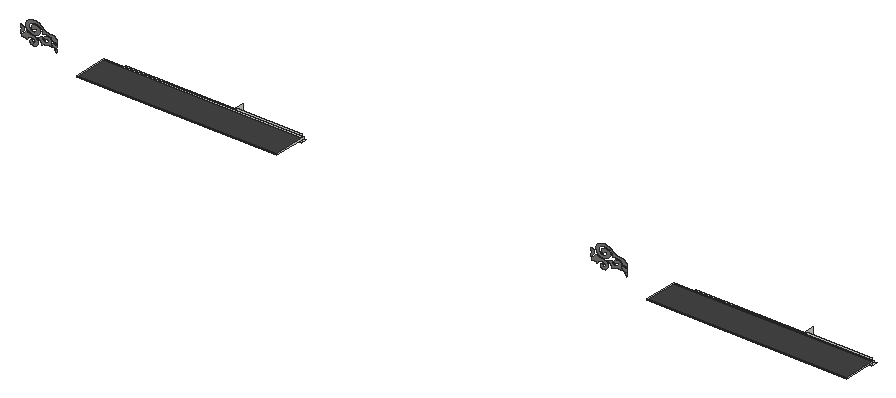
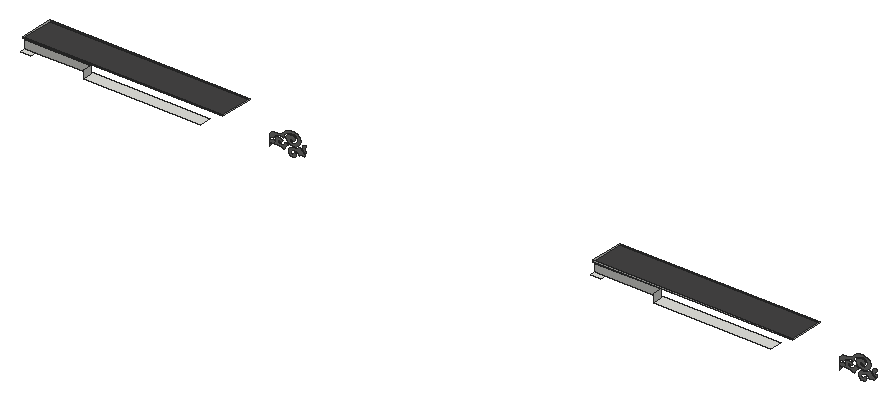
# SketchUp Ruby script. Lengths in inches.
U = 1.inch
M = Sketchup.active_model
def pt(a) = Geom::Point3d.new(a.map { |v| v * U })
def face(e, loops, mat)
  f = e.add_face(loops[0].map { |a| pt(a) })
  loops[1..].each { |l| e.add_face(l.map { |a| pt(a) }).erase! }
  f.material = f.back_material = mat if mat
  f
end
# faces: each face lists its corners as indices into pts; further lists are holes
def faces(e, pts, list, mat = nil) = list.each { |f| face(e, (f[0].is_a?(Array) ? f : [f]).map { |l| l.map { |i| pts[i] } }, mat) }
# xy, xz, yz: faces in a plane at the given z, y or x. An outline is a flat list of corners, or four numbers for a rectangle; further outlines are holes
def ring(l) = l.size == 4 ? [[l[0], l[1]], [l[2], l[1]], [l[2], l[3]], [l[0], l[3]]] : l.each_slice(2).to_a
def flat(e, list, mat, &to3) = list.each { |f| face(e, (f[0].is_a?(Array) ? f : [f]).map { |l| ring(l).map { |u, v| to3.(u, v) } }, mat) }
def xy(e, z, list, mat = nil) = flat(e, list, mat) { |x, y| [x, y, z] }
def xz(e, y, list, mat = nil) = flat(e, list, mat) { |x, z| [x, y, z] }
def yz(e, x, list, mat = nil) = flat(e, list, mat) { |y, z| [x, y, z] }
def lines(e, pts, list) = list.each { |a, b| e.add_line(pt(pts[a]), pt(pts[b])) }
# prism: a flat outline (further loops are holes) pulled along v
def prism(e, loops, v, mat = nil)
  f = face(e, loops, mat); d = Geom::Vector3d.new(v.map { |x| x * U })
  f.pushpull(f.normal.samedirection?(d) ? d.length : -d.length)
end
def box(e, o, s, mat = nil) = prism(e, [[o, [o[0] + s[0], o[1], o[2]], [o[0] + s[0], o[1] + s[1], o[2]], [o[0], o[1] + s[1], o[2]]]], [0, 0, s[2]], mat)
def at(x, y, z, deg = 0) = Geom::Transformation.translation(pt([x, y, z])) * Geom::Transformation.rotation(ORIGIN, Z_AXIS, deg.degrees)
def axes(o, x, y, z) = Geom::Transformation.new([*x, 0, *y, 0, *z, 0, *pt(o).to_a, 1])
def part(name) = M.definitions.add(name)
# library, detail: a bought-in or finely detailed component or shape, given as its bounding box
def library(name, o, s) = part(name).tap { |d| box(d.entities, o, s) }
def detail(e, o, s) = box(e.add_group.entities, o, s)
def put(e, d, t, mat = nil) = e.add_instance(d, t).tap { |i| i.material = mat if mat }
def group(e, t, mat = nil) = e.add_group.tap { |g| g.transformation = t; g.material = mat if mat }.entities
root = M.entities
M.materials.add("[0043_SaddleBrown]4").color = [124, 123, 122]
M.materials.add("[Granite Dark Gray]").color = [69, 68, 68]
xy(root,251.46,[[578.37,589.17,578.37,616,835.39,616,835.39,595.44,956.36,595.44,956.36,589.17],[1829,589.17,1829,616,2086.01,616,2086.01,595.44,2206.98,595.44,2206.98,589.17],[956.36,595.44,979.42,608.75],[2206.98,595.44,2230.05,608.75]])
xy(root,265.8125,[[551.76,515.0625,990.19,589.17],[1802.38,515.0625,2240.81,589.17]],"[Granite Dark Gray]")
xz(root,515.0625,[[551.76,265.8125,990.19,268.4375],[1802.38,265.8125,2240.81,268.4375]],"[Granite Dark Gray]")
xz(root,589.17,[[551.76,265.8125,990.19,268.4375],[1802.38,265.8125,2240.81,268.4375]])
xz(root,589.17,[[397.84,240.53,396.24,240.59,394.6875,240.89,393.26,241.42,392.02,242.16,391.02,243.07,390.31,244.1,389.91,245.23,389.86,246.39,389.92,246.75,390.03,247.1,390.19,247.44,390.4,247.77,390.66,248.09,390.96,248.38,391.3,248.64,391.67,248.89,392.08,249.1,392.52,249.28,392.98,249.43,393.46,249.54,393.54,249.03,393.66,248.52,393.82,248.02,394.03,247.53,394.27,247.05,394.55,246.58,394.87,246.12,395.23,245.67,395.62,245.24,396.04,244.83,396.5,244.4375,396.99,244.07,397.92,244.4,398.77,244.84,399.52,245.37,400.15,245.97,400.64,246.64,400.98,247.35,401.17,248.09,401.19,248.85,401.05,249.59,400.76,250.32,400.32,251,399.73,251.625,398.89,252.57,397.82,253.38,396.57,254.04,395.17,254.51,393.67,254.8,392.12,254.88,390.58,254.75,389.09,254.42,387.72,253.9,386.51,253.2,385.49,252.35,384.71,251.39,384.49,251.13,384.29,250.86,384.1,250.6,383.92,250.32,383.75,250.05,383.6,249.77,383.46,249.48,383.33,249.2,383.11,248.62,383.02,248.32,382.95,248.02,382.26,248.6875,381.46,249.28,380.56,249.8,379.58,250.24,378.53,250.58,377.4375,250.83,376.3,250.97,375.16,251.02,374.01,250.96,372.88,250.8,371.79,250.54,370.75,250.18,370.97,250.49,371.16,250.81,371.32,251.13,371.46,251.47,371.58,251.8,371.66,252.14,371.72,252.49,371.75,252.83,371.76,253.18,371.73,253.53,371.68,253.875,371.6,254.22,372.75,254.84,373.84,255.51,374.9,256.21,375.9,256.95,376.86,257.73,377.76,258.53,378.61,259.37,379.4,260.23,380.13,261.12,380.8,262.04,381.41,262.97,381.96,263.93,382.57,263.15,383.29,262.41,384.1,261.73,385.01,261.12,386,260.57,387.0625,260.1,388.19,259.71,389.36,259.41,390.57,259.19,391.8,259.0625,393.04,259.03,394.29,259.08,396.7,258.68,398.99,257.98,401.07,257,402.875,255.77,404.36,254.34,405.48,252.74,406.19,251.03,406.48,249.25,406.33,247.46,405.76,245.72,404.77,244.08,403.4,242.59,402.27,241.76,400.93,241.125,399.43,240.71],[1648.47,240.53,1646.86,240.59,1645.3125,240.89,1643.89,241.42,1642.64,242.16,1641.65,243.07,1640.93,244.1,1640.54,245.23,1640.48,246.39,1640.54,246.75,1640.65,247.1,1640.82,247.44,1641.03,247.77,1641.28,248.09,1641.58,248.38,1641.92,248.64,1642.3,248.89,1642.71,249.1,1643.14,249.28,1643.6,249.43,1644.08,249.54,1644.16,249.03,1644.29,248.52,1644.45,248.02,1644.65,247.53,1644.9,247.05,1645.18,246.58,1645.5,246.12,1645.85,245.67,1646.24,245.24,1646.67,244.83,1647.125,244.4375,1647.61,244.07,1648.55,244.4,1649.4,244.84,1650.15,245.37,1650.77,245.97,1651.26,246.64,1651.61,247.35,1651.79,248.09,1651.82,248.85,1651.68,249.59,1651.39,250.32,1650.94,251,1650.35,251.625,1649.52,252.57,1648.45,253.38,1647.19,254.04,1645.79,254.51,1644.29,254.8,1642.74,254.88,1641.2,254.75,1639.72,254.42,1638.35,253.9,1637.13,253.2,1636.12,252.35,1635.33,251.39,1635.12,251.13,1634.92,250.86,1634.72,250.6,1634.54,250.32,1634.38,250.05,1634.22,249.77,1634.08,249.48,1633.96,249.2,1633.84,248.91,1633.74,248.62,1633.65,248.32,1633.58,248.02,1632.88,248.6875,1632.08,249.28,1631.19,249.8,1630.21,250.24,1629.16,250.58,1628.0625,250.83,1626.93,250.97,1625.78,251.02,1624.63,250.96,1623.5,250.8,1622.41,250.54,1621.375,250.18,1621.59,250.49,1621.78,250.81,1621.95,251.13,1622.09,251.47,1622.2,251.8,1622.29,252.14,1622.35,252.49,1622.38,252.83,1622.38,253.18,1622.36,253.53,1622.31,253.875,1622.23,254.22,1623.37,254.84,1624.47,255.51,1625.52,256.21,1626.53,256.95,1627.48,257.73,1628.38,258.53,1629.23,259.37,1630.02,260.23,1630.76,261.12,1631.43,262.04,1632.04,262.97,1632.59,263.93,1633.2,263.15,1633.91,262.41,1634.73,261.73,1635.64,261.12,1636.625,260.57,1637.6875,260.1,1638.81,259.71,1639.98,259.41,1641.19,259.19,1642.42,259.0625,1643.67,259.03,1644.91,259.08,1647.33,258.68,1649.61,257.98,1651.69,257,1653.5,255.77,1654.99,254.34,1656.1,252.74,1656.82,251.03,1657.1,249.25,1656.96,247.46,1656.38,245.72,1655.39,244.08,1654.02,242.59,1652.9,241.76,1651.55,241.125,1650.06,240.71],[448.37,243.61,448.09,244.05,447.79,244.49,447.49,244.92,447.17,245.34,446.84,245.77,446.5,246.18,446.15,246.6,445.79,247,445.03,247.8,444.63,248.1875,444.22,248.57,444.5,248.76,444.79,248.9375,445.1,249.1,445.43,249.24,445.77,249.36,446.12,249.47,446.48,249.56,446.85,249.625,447.22,249.68,447.6,249.71,447.98,249.72,448.37,249.7],[1698.99,243.61,1698.71,244.05,1698.42,244.49,1698.11,244.92,1697.8,245.34,1697.47,245.77,1697.13,246.18,1696.78,246.6,1696.04,247.4,1695.65,247.8,1695.25,248.1875,1694.85,248.57,1695.12,248.76,1695.42,248.9375,1695.73,249.1,1696.05,249.24,1696.39,249.36,1696.74,249.47,1697.1,249.56,1697.47,249.625,1697.85,249.68,1698.23,249.71,1698.61,249.72,1698.99,249.7],[415.32,248.92,415.21,249.99,414.98,251.04,414.64,252.09,414.19,253.11,413.64,254.1,412.99,255.07,412.24,255.99,411.39,256.87,410.46,257.7,409.4375,258.48,408.34,259.21,407.17,259.87,407.79,260.07,409.01,260.51,409.61,260.74,410.2,260.97,410.79,261.22,411.37,261.48,411.94,261.74,412.5,262.01,413.0625,262.29,413.61,262.58,414.15,262.88,414.26,261.48,414.78,260.125,415.7,258.89,416.98,257.82,418.54,256.98,420.32,256.41,422.22,256.13,424.17,256.15,426.07,256.48,427.82,257.1,429.34,257.97,430.56,259.07,430.6,259.41,430.62,259.75,430.62,260.43,430.56,261.11,430.51,261.45,430.44,261.79,430.36,262.12,430.27,262.46,430.17,262.79,430.04,263.12,429.45,263.3,428.82,263.42,428.18,263.46,427.53,263.43,426.9,263.32,426.3,263.15,425.75,262.9,425.25,262.6,424.83,262.24,424.5,261.85,424.25,261.41,424.11,260.96,423.7,261.08,423.3125,261.23,422.93,261.39,422.57,261.57,422.22,261.77,421.89,261.98,421.58,262.2,421.28,262.44,421.01,262.69,420.77,262.96,420.54,263.23,420.34,263.51,420.93,264.63,421.82,265.64,422.98,266.5,424.36,267.17,425.89,267.62,427.53,267.84,429.1875,267.81,430.81,267.54,432.3125,267.03,433.64,266.3125,434.74,265.42,435.56,264.375,435,263.4375,434.55,262.46,434.23,261.47,434.03,260.45,433.95,259.43,434,258.41,434.18,257.39,434.48,256.39,434.9,255.41,435.44,254.47,436.1,253.56,436.86,252.69,434.98,252.81,433.1,252.84,431.21,252.8,429.34,252.67,427.47,252.47,425.63,252.1875,423.81,251.83,422.02,251.39,420.28,250.88,418.57,250.3,416.92,249.64],
  [1665.95,248.92,1665.83,249.99,1665.6,251.04,1665.26,252.09,1664.82,253.11,1664.26,254.1,1663.61,255.07,1662.86,255.99,1662.02,256.87,1661.08,257.7,1660.0625,258.48,1658.97,259.21,1657.8,259.87,1658.42,260.07,1659.64,260.51,1660.23,260.74,1660.83,260.97,1661.41,261.22,1661.99,261.48,1662.56,261.74,1663.13,262.01,1663.6875,262.29,1664.23,262.58,1664.77,262.88,1664.88,261.48,1665.41,260.125,1666.33,258.89,1667.6,257.82,1669.16,256.98,1670.94,256.41,1672.85,256.13,1674.8,256.15,1676.69,256.48,1678.44,257.1,1679.96,257.97,1681.18,259.07,1681.22,259.41,1681.24,259.75,1681.25,260.09,1681.24,260.43,1681.22,260.77,1681.18,261.11,1681.13,261.45,1681.07,261.79,1680.99,262.12,1680.9,262.46,1680.79,262.79,1680.67,263.12,1680.08,263.3,1679.45,263.42,1678.8,263.46,1678.16,263.43,1677.52,263.32,1676.92,263.15,1676.37,262.9,1675.88,262.6,1675.46,262.24,1675.12,261.85,1674.88,261.41,1674.73,260.96,1674.33,261.08,1673.9375,261.23,1673.56,261.39,1673.19,261.57,1672.84,261.77,1672.51,261.98,1672.2,262.2,1671.91,262.44,1671.64,262.69,1671.39,262.96,1671.17,263.23,1670.97,263.51,1671.55,264.63,1672.44,265.64,1673.6,266.5,1674.98,267.17,1676.52,267.62,1678.15,267.84,1679.8125,267.81,1681.43,267.54,1682.9375,267.03,1684.27,266.3125,1685.37,265.42,1686.19,264.375,1685.625,263.4375,1685.18,262.46,1684.86,261.47,1684.65,260.45,1684.58,259.43,1684.63,258.41,1684.81,257.39,1685.11,256.39,1685.53,255.41,1686.07,254.47,1686.72,253.56,1687.49,252.69,1685.61,252.81,1683.72,252.84,1681.84,252.8,1679.96,252.67,1678.1,252.47,1676.25,252.1875,1674.43,251.83,1672.65,251.39,1670.9,250.88,1669.2,250.3,1667.55,249.64],[444.15,252.36,443.05,252.47,441.99,252.71,440.99,253.0625,440.09,253.53,439.3,254.09,438.64,254.73,438.13,255.44,437.79,256.2,437.53,256.55,437.375,256.93,437.32,257.32,437.37,257.71,437.53,258.08,437.78,258.43,438.12,258.74,438.53,258.99,439.01,259.18,439.53,259.31,440.07,259.36,440.61,259.33,441.07,259.26,441.53,259.16,441.96,259.03,442.38,258.87,442.78,258.6875,443.16,258.48,443.51,258.25,443.83,257.99,444.11,257.72,444.36,257.43,444.58,257.13,444.76,256.8125,445.1,256.95,445.4375,257.09,445.77,257.24,446.09,257.4,446.41,257.57,446.72,257.75,447.02,257.93,447.31,258.125,447.59,258.32,447.86,258.53,448.12,258.74,448.37,258.96,448.37,253.18,447.39,252.79,446.35,252.53,445.26,252.38],[1694.77,252.36,1693.67,252.47,1692.61,252.71,1691.62,253.0625,1690.71,253.53,1689.92,254.09,1689.26,254.73,1688.76,255.44,1688.41,256.2,1688.16,256.55,1688,256.93,1687.95,257.32,1688,257.71,1688.15,258.08,1688.4,258.43,1688.74,258.74,1689.16,258.99,1689.63,259.18,1690.15,259.31,1690.69,259.36,1691.23,259.33,1691.7,259.26,1692.15,259.16,1692.59,259.03,1693.01,258.87,1693.41,258.6875,1693.78,258.48,1694.13,258.25,1694.45,257.99,1694.74,257.72,1694.99,257.43,1695.2,257.13,1695.38,256.8125,1695.73,256.95,1696.0625,257.09,1696.4,257.24,1696.72,257.4,1697.03,257.57,1697.34,257.75,1697.64,257.93,1697.93,258.125,1698.21,258.32,1698.48,258.53,1698.74,258.74,1698.99,258.96,1698.99,253.18,1698.02,252.79,1696.97,252.53,1695.88,252.38],[367.98,255.94,367.98,260.6875,369.06,261.02,370.02,261.5,370.82,262.125,371.42,262.86,371.79,263.66,371.92,264.5,371.79,265.35,371.42,266.15,370.82,266.88,370.02,267.51,369.06,267.99,367.98,268.32,367.98,272.35,369.22,272.27,370.44,272.07,371.61,271.73,372.68,271.26,373.65,270.6875,374.49,270.02,375.17,269.26,375.6875,268.44,376.03,267.56,376.18,266.67,376.14,265.76,375.91,264.875,375.5625,264.01,375.15,263.17,374.68,262.33,374.15,261.52,373.56,260.73,372.91,259.96,372.22,259.22,371.46,258.5,370.66,257.8125,369.8125,257.16,368.92,256.53],[1618.6,255.94,1618.6,260.6875,1619.68,261.02,1620.65,261.5,1621.45,262.125,1622.05,262.86,1622.42,263.66,1622.54,264.5,1622.42,265.35,1622.05,266.15,1621.45,266.88,1620.65,267.51,1619.68,267.99,1618.6,268.32,1618.6,272.35,1619.85,272.27,1621.07,272.07,1622.23,271.73,1623.31,271.26,1624.27,270.6875,1625.11,270.02,1625.79,269.26,1626.3125,268.44,1626.65,267.56,1626.8,266.67,1626.76,265.76,1626.54,264.875,1626.1875,264.01,1625.78,263.17,1625.3,262.33,1624.77,261.52,1624.18,260.73,1623.54,259.96,1622.84,259.22,1622.09,258.5,1621.29,257.8125,1620.4375,257.16,1619.54,256.53],
  [448.37,260.7,448,261.39,447.5,262.04,446.88,262.64,446.15,263.17,445.33,263.61,444.43,263.97,443.46,264.24,442.45,264.41,441.43,264.47,440.4,264.42,439.38,264.28,438.41,264.03,437.97,265.63,437.15,267.16,435.99,268.56,434.51,269.79,432.76,270.83,430.79,271.64,428.66,272.19,426.43,272.47,424.16,272.48,421.93,272.2,419.79,271.65,417.82,270.85,417.76,272.875,417.29,274.87,416.43,276.79,415.1875,278.6,413.6,280.27,411.68,281.75,409.5,283.01,407.08,284.03,404.48,284.79,401.75,285.27,398.96,285.46,396.16,285.35,393.71,284.63,391.5,283.58,389.61,282.24,388.11,280.66,387.07,278.9,386.51,277.03,386.47,275.12,386.9375,273.24,387.9,271.46,389.32,269.85,391.15,268.46,393.3125,267.36,394.71,266.91,396.2,266.68,397.72,266.68,399.22,266.89,400.62,267.33,401.87,267.96,402.92,268.76,403.71,269.69,404.23,270.73,404.44,271.82,404.35,272.91,403.94,273.97,403.66,274.36,403.29,274.7,402.82,274.98,402.29,275.19,401.71,275.32,401.11,275.37,400.5,275.32,399.92,275.19,399.39,274.98,398.93,274.7,398.55,274.36,398.27,273.97,398.14,273.75,397.98,273.53,397.79,273.32,397.58,273.13,397.35,272.95,397.1,272.78,396.83,272.625,396.55,272.49,396.25,272.37,395.93,272.27,395.61,272.1875,395.28,272.125,394.7,272.37,394.17,272.67,393.69,273.01,393.27,273.39,392.91,273.8,392.64,274.25,392.43,274.71,392.3125,275.1875,392.27,275.67,392.32,276.16,392.44,276.64,392.65,277.1,393.04,277.72,393.52,278.31,394.08,278.86,394.73,279.36,395.44,279.81,396.22,280.2,397.05,280.52,397.92,280.79,398.83,280.98,399.76,281.1,400.7,281.15,401.65,281.125,403.14,280.95,404.59,280.64,405.97,280.19,407.25,279.62,408.41,278.92,409.44,278.12,410.3,277.23,411,276.26,411.51,275.24,411.82,274.17,411.9375,273.09,411.85,272,411.25,270.37,410.32,268.8125,409.1,267.37,407.61,266.06,405.88,264.92,403.9375,263.97,401.83,263.23,399.6,262.71,397.28,262.42,394.9375,262.375,392.6,262.57,390.34,263,388.14,264.08,386.16,265.36,384.42,266.82,382.97,268.42,381.81,270.15,380.97,271.97,380.46,273.85,380.3,275.77,380.48,277.68,381,279.5625,381.86,281.375,383.04,283.1,384.84,284.97,387.06,286.6,389.63,287.93,392.47,288.93,395.51,289.57,398.65,289.83,401.81,289.71,404.89,289.2,407.8125,288.32,410.49,287.1,412.84,285.58,414.79,283.78,415.33,283.04,415.92,282.32,416.56,281.61,417.24,280.93,417.97,280.27,418.73,279.64,419.54,279.04,420.39,278.46,421.27,277.91,422.19,277.4,423.14,276.91,424.125,276.46,425.43,276.01,426.76,275.62,428.125,275.28,429.51,274.99,430.92,274.76,432.34,274.59,433.77,274.47,435.21,274.41,436.65,274.41,438.09,274.47,439.53,274.58,440.95,274.75,442.07,273.47,442.65,272.84,443.24,272.22,443.85,271.6,444.46,270.99,445.08,270.38,446.36,269.18,447.02,268.6,447.6875,268.01,448.37,267.4375],[1698.99,260.7,1698.625,261.39,1698.125,262.04,1697.51,262.64,1696.78,263.17,1695.95,263.61,1695.05,263.97,1694.09,264.24,1693.08,264.41,1692.05,264.47,1691.02,264.42,1690.01,264.28,1689.03,264.03,1688.59,265.63,1687.78,267.16,1686.61,268.56,1685.13,269.79,1683.38,270.83,1681.41,271.64,1679.28,272.19,1677.05,272.47,1674.79,272.48,1672.55,272.2,1670.42,271.65,1668.45,270.85,1668.38,272.875,1667.92,274.87,1667.05,276.79,1665.8125,278.6,1664.22,280.27,1662.31,281.75,1660.12,283.01,1657.7,284.03,1655.1,284.79,1652.38,285.27,1649.59,285.46,1646.79,285.35,1644.34,284.63,1642.12,283.58,1640.23,282.24,1638.74,280.66,1637.69,278.9,1637.14,277.03,1637.09,275.12,1637.5625,273.24,1638.53,271.46,1639.95,269.85,1641.77,268.46,1643.9375,267.36,1645.33,266.91,1646.82,266.68,1648.35,266.68,1649.84,266.89,1651.24,267.33,1652.5,267.96,1653.54,268.76,1654.34,269.69,1654.86,270.73,1655.07,271.82,1654.97,272.91,1654.56,273.97,1654.29,274.36,1653.91,274.7,1653.45,274.98,1652.91,275.19,1652.34,275.32,1651.73,275.37,1651.13,275.32,1650.55,275.19,1650.02,274.98,1649.55,274.7,1649.18,274.36,1648.9,273.97,1648.76,273.75,1648.6,273.53,1648.41,273.32,1648.2,273.13,1647.97,272.95,1647.72,272.78,1647.46,272.625,1647.17,272.49,1646.87,272.37,1646.56,272.27,1646.24,272.1875,1645.91,272.125,1645.33,272.37,1644.79,272.67,1644.31,273.01,1643.89,273.39,1643.54,273.8,1643.26,274.25,1643.06,274.71,1642.9375,275.1875,1642.9,275.67,1642.94,276.16,1643.07,276.64,1643.27,277.1,1643.66,277.72,1644.14,278.31,1644.71,278.86,1645.35,279.36,1646.07,279.81,1646.84,280.2,1647.67,280.52,1648.55,280.79,1649.45,280.98,1650.38,281.1,1651.33,281.15,1652.27,281.125,1653.77,280.95,1655.21,280.64,1656.59,280.19,1657.87,279.62,1659.04,278.92,1660.06,278.12,1660.93,277.23,1661.62,276.26,1662.13,275.24,1662.45,274.17,1662.5625,273.09,1662.48,272,1661.87,270.37,1660.95,268.8125,1659.73,267.37,1658.24,266.06,1656.5,264.92,1654.5625,263.97,1652.45,263.23,1650.22,262.71,1647.91,262.42,1645.5625,262.375,1643.23,262.57,1640.96,263,1638.77,264.08,1636.78,265.36,1635.05,266.82,1633.59,268.42,1632.43,270.15,1631.59,271.97,1631.09,273.85,1630.92,275.77,1631.1,277.68,1631.63,279.5625,1632.49,281.375,1633.66,283.1,1635.47,284.97,1637.69,286.6,1640.25,287.93,1643.1,288.93,1646.13,289.57,1649.27,289.83,1652.43,289.71,1655.52,289.2,1658.4375,288.32,1661.11,287.1,1663.46,285.58,1665.42,283.78,1665.96,283.04,1666.55,282.32,1667.18,281.61,1667.87,280.93,1668.59,280.27,1669.36,279.64,1670.17,279.04,1671.01,278.46,1671.9,277.91,1672.82,277.4,1673.77,276.91,1674.75,276.46,1676.05,276.01,1677.39,275.62,1678.75,275.28,1680.14,274.99,1681.54,274.76,1682.96,274.59,1684.4,274.47,1685.84,274.41,1687.28,274.41,1688.72,274.47,1690.15,274.58,1691.58,274.75,1692.13,274.11,1692.7,273.47,1693.28,272.84,1693.87,272.22,1694.47,271.6,1695.08,270.99,1695.71,270.38,1696.34,269.78,1696.99,269.18,1697.65,268.6,1698.3125,268.01,1698.99,267.4375]],"[0043_SaddleBrown]4")
xz(root,595.44,[[835.39,251.46,979.42,268.4375],[2086.01,251.46,2230.05,268.4375]])
yz(root,551.76,[[515.0625,265.8125,589.17,268.4375]])
yz(root,835.39,[[595.44,251.46,616,268.4375]])
yz(root,990.19,[[515.0625,265.8125,589.17,268.4375]])
yz(root,1802.38,[[515.0625,265.8125,589.17,268.4375]])
yz(root,2086.01,[[595.44,251.46,616,268.4375]])
yz(root,2240.81,[[515.0625,265.8125,589.17,268.4375]])
